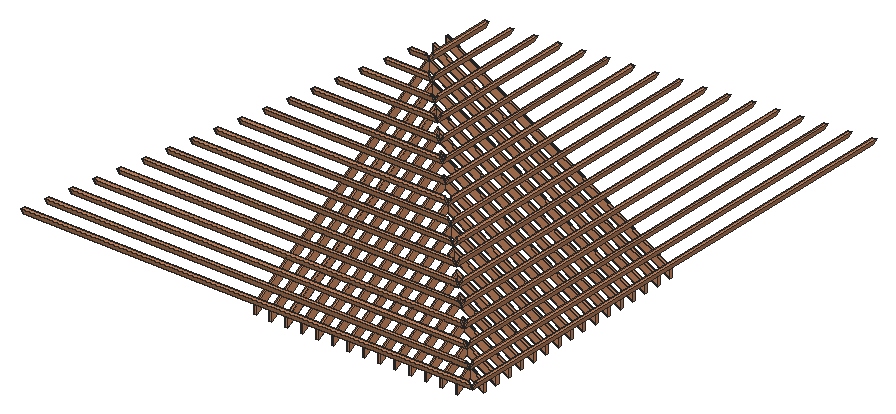
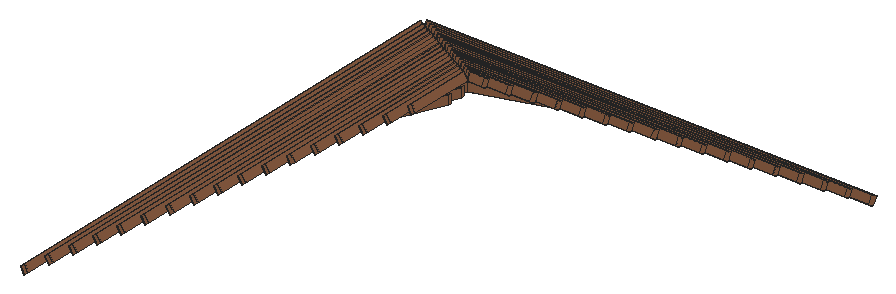
# SketchUp Ruby script. Lengths in millimetres.
U = 1.mm
M = Sketchup.active_model
def pt(a) = Geom::Point3d.new(a.map { |v| v * U })
def face(e, loops, mat)
  f = e.add_face(loops[0].map { |a| pt(a) })
  loops[1..].each { |l| e.add_face(l.map { |a| pt(a) }).erase! }
  f.material = f.back_material = mat if mat
  f
end
# faces: each face lists its corners as indices into pts; further lists are holes
def faces(e, pts, list, mat = nil) = list.each { |f| face(e, (f[0].is_a?(Array) ? f : [f]).map { |l| l.map { |i| pts[i] } }, mat) }
# xy, xz, yz: faces in a plane at the given z, y or x. An outline is a flat list of corners, or four numbers for a rectangle; further outlines are holes
def ring(l) = l.size == 4 ? [[l[0], l[1]], [l[2], l[1]], [l[2], l[3]], [l[0], l[3]]] : l.each_slice(2).to_a
def flat(e, list, mat, &to3) = list.each { |f| face(e, (f[0].is_a?(Array) ? f : [f]).map { |l| ring(l).map { |u, v| to3.(u, v) } }, mat) }
def xy(e, z, list, mat = nil) = flat(e, list, mat) { |x, y| [x, y, z] }
def xz(e, y, list, mat = nil) = flat(e, list, mat) { |x, z| [x, y, z] }
def yz(e, x, list, mat = nil) = flat(e, list, mat) { |y, z| [x, y, z] }
def lines(e, pts, list) = list.each { |a, b| e.add_line(pt(pts[a]), pt(pts[b])) }
# prism: a flat outline (further loops are holes) pulled along v
def prism(e, loops, v, mat = nil)
  f = face(e, loops, mat); d = Geom::Vector3d.new(v.map { |x| x * U })
  f.pushpull(f.normal.samedirection?(d) ? d.length : -d.length)
end
def box(e, o, s, mat = nil) = prism(e, [[o, [o[0] + s[0], o[1], o[2]], [o[0] + s[0], o[1] + s[1], o[2]], [o[0], o[1] + s[1], o[2]]]], [0, 0, s[2]], mat)
def at(x, y, z, deg = 0) = Geom::Transformation.translation(pt([x, y, z])) * Geom::Transformation.rotation(ORIGIN, Z_AXIS, deg.degrees)
def axes(o, x, y, z) = Geom::Transformation.new([*x, 0, *y, 0, *z, 0, *pt(o).to_a, 1])
def part(name) = M.definitions.add(name)
# library, detail: a bought-in or finely detailed component or shape, given as its bounding box
def library(name, o, s) = part(name).tap { |d| box(d.entities, o, s) }
def detail(e, o, s) = box(e.add_group.entities, o, s)
def put(e, d, t, mat = nil) = e.add_instance(d, t).tap { |i| i.material = mat if mat }
def group(e, t, mat = nil) = e.add_group.tap { |g| g.transformation = t; g.material = mat if mat }.entities
root = M.entities
M.materials.add("[Wood Veneer 02]").color = [190, 128, 91]
c1 = part("Group243\#1")
prism(c1.entities,[[[4410,-2546.1,0],[-4410,-2546.1,0],[-4365.8,-2495.1,0],[4365.8,-2495.1,0]]],[0,0,152])
c2 = part("Group244\#1")
prism(c2.entities,[[[4145.9,-2241.1,0],[-4145.9,-2241.1,0],[-4101.7,-2190.1,0],[4101.7,-2190.1,0]]],[0,0,152])
c3 = part("Group245\#1")
prism(c3.entities,[[[3881.7,-1936.1,0],[-3881.7,-1936.1,0],[-3837.6,-1885.1,0],[3837.6,-1885.1,0]]],[0,0,152])
c4 = part("Group246\#1")
prism(c4.entities,[[[-3573.4,-1580.1,0],[3573.4,-1580.1,0],[3617.6,-1631.1,0],[-3617.6,-1631.1,0]]],[0,0,152])
c5 = part("Group247\#1")
prism(c5.entities,[[[-3309.3,-1275.1,0],[3309.3,-1275.1,0],[3353.4,-1326.1,0],[-3353.4,-1326.1,0]]],[0,0,152])
c6 = part("Group248\#1")
prism(c6.entities,[[[3089.3,-1021.1,0],[-3089.3,-1021.1,0],[-3045.1,-970.1,0],[3045.1,-970.1,0]]],[0,0,152])
c7 = part("Group249\#1")
prism(c7.entities,[[[-2781,-665.1,0],[2781,-665.1,0],[2825.2,-716.1,0],[-2825.2,-716.1,0]]],[0,0,152])
c8 = part("Group250\#1")
prism(c8.entities,[[[-2516.9,-360.1,0],[2516.9,-360.1,0],[2561,-411.1,0],[-2561,-411.1,0]]],[0,0,152])
c9 = part("Group251\#1")
prism(c9.entities,[[[-2252.7,-55.1,0],[2252.7,-55.1,0],[2296.9,-106.1,0],[-2296.9,-106.1,0]]],[0,0,152])
c10 = part("Group252\#1")
prism(c10.entities,[[[2032.8,198.9,0],[-2032.8,198.9,0],[-1988.6,249.9,0],[1988.6,249.9,0]]],[0,0,152])
c11 = part("Group253\#1")
prism(c11.entities,[[[1768.6,503.9,0],[-1768.6,503.9,0],[-1724.5,554.9,0],[1724.5,554.9,0]]],[0,0,152])
c12 = part("Group254\#1")
prism(c12.entities,[[[1504.5,808.9,0],[-1504.5,808.9,0],[-1460.3,859.9,0],[1460.3,859.9,0]]],[0,0,152])
c13 = part("Group255\#1")
prism(c13.entities,[[[-1196.2,1164.9,0],[1196.2,1164.9,0],[1240.3,1113.9,0],[-1240.3,1113.9,0]]],[0,0,152])
c14 = part("Group256\#1")
prism(c14.entities,[[[-932,1469.9,0],[932,1469.9,0],[976.2,1418.9,0],[-976.2,1418.9,0]]],[0,0,152])
c15 = part("Group257\#1")
prism(c15.entities,[[[712.1,1723.9,0],[-712.1,1723.9,0],[-667.9,1774.9,0],[667.9,1774.9,0]]],[0,0,152])
c16 = part("Group258\#1")
prism(c16.entities,[[[447.9,2028.9,0],[-447.9,2028.9,0],[-403.8,2079.9,0],[403.8,2079.9,0]]],[0,0,152])
c17 = part("Group259\#1")
prism(c17.entities,[[[183.8,2333.9,0],[-183.8,2333.9,0],[-139.6,2384.9,0],[139.6,2384.9,0]]],[0,0,152])
c18 = part("Group241\#2")
put(c18.entities,c1,at(0,0,0))
put(c18.entities,c2,at(0,0,0))
put(c18.entities,c3,at(0,0,0))
put(c18.entities,c4,at(0,0,0))
put(c18.entities,c5,at(0,0,0))
put(c18.entities,c6,at(0,0,0))
put(c18.entities,c7,at(0,0,0))
put(c18.entities,c8,at(0,0,0))
put(c18.entities,c9,at(0,0,0))
put(c18.entities,c10,at(0,0,0))
put(c18.entities,c11,at(0,0,0))
put(c18.entities,c12,at(0,0,0))
put(c18.entities,c13,at(0,0,0))
put(c18.entities,c14,at(0,0,0))
put(c18.entities,c15,at(0,0,0))
put(c18.entities,c16,at(0,0,0))
put(c18.entities,c17,at(0,0,0))
c19 = part("Group241\#1")
xy(c19.entities,0,[[-4960,-4295.5,-4901.1,-4244.5,0,-4244.5,0,-4295.5]])
xy(c19.entities,152,[[-5047.8,-4295.5,-87.8,-4295.5,-87.8,-4244.5,-4988.9,-4244.5]])
xz(c19.entities,-4295.5,[[-4960,0,0,0,-87.8,152,-5047.8,152]])
xz(c19.entities,-4244.5,[[-4901.1,0,-4988.9,152,-87.8,152,0,0]])
p = [[-4901.1,-4244.5,0],[-4960,-4295.5,0],[-5047.8,-4295.5,152],[-4988.9,-4244.5,152],[0,-4295.5,0],[0,-4244.5,0],
  [-87.8,-4244.5,152],[-87.8,-4295.5,152]]
faces(c19.entities,p,[[0,1,2,3],[4,5,6,7]])
c20 = part("Group239\#1")
xy(c20.entities,0,[[-4607.8,-3990.5,-4548.9,-3939.5,0,-3939.5,0,-3990.5]])
xy(c20.entities,152,[[-4695.6,-3990.5,-87.8,-3990.5,-87.8,-3939.5,-4636.7,-3939.5]])
xz(c20.entities,-3990.5,[[-4607.8,0,0,0,-87.8,152,-4695.6,152]])
xz(c20.entities,-3939.5,[[-4548.9,0,-4636.7,152,-87.8,152,0,0]])
p = [[-4636.7,-3939.5,152],[-4548.9,-3939.5,0],[-4607.8,-3990.5,0],[-4695.6,-3990.5,152],[0,-3939.5,0],[-87.8,-3939.5,152],
  [-87.8,-3990.5,152],[0,-3990.5,0]]
faces(c20.entities,p,[[0,1,2,3],[4,5,6,7]])
c21 = part("Group237\#1")
xy(c21.entities,0,[[-4255.6,-3685.5,-4196.8,-3634.5,0,-3634.5,0,-3685.5]])
xy(c21.entities,152,[[-4343.4,-3685.5,-87.8,-3685.5,-87.8,-3634.5,-4284.5,-3634.5]])
xz(c21.entities,-3685.5,[[-4255.6,0,0,0,-87.8,152,-4343.4,152]])
xz(c21.entities,-3634.5,[[-4196.8,0,-4284.5,152,-87.8,152,0,0]])
p = [[-4284.5,-3634.5,152],[-4196.8,-3634.5,0],[-4255.6,-3685.5,0],[-4343.4,-3685.5,152],[0,-3634.5,0],[-87.8,-3634.5,152],
  [-87.8,-3685.5,152],[0,-3685.5,0]]
faces(c21.entities,p,[[0,1,2,3],[4,5,6,7]])
c22 = part("Group235\#1")
xy(c22.entities,0,[[-3903.5,-3380.5,-3844.6,-3329.5,0,-3329.5,0,-3380.5]])
xy(c22.entities,152,[[-3991.2,-3380.5,-87.8,-3380.5,-87.8,-3329.5,-3932.3,-3329.5]])
xz(c22.entities,-3380.5,[[-3903.5,0,0,0,-87.8,152,-3991.2,152]])
xz(c22.entities,-3329.5,[[-3844.6,0,-3932.3,152,-87.8,152,0,0]])
p = [[-3991.2,-3380.5,152],[-3932.3,-3329.5,152],[-3844.6,-3329.5,0],[-3903.5,-3380.5,0],[-87.8,-3329.5,152],[-87.8,-3380.5,152],
  [0,-3380.5,0],[0,-3329.5,0]]
faces(c22.entities,p,[[0,1,2,3],[4,5,6,7]])
c23 = part("Group233\#1")
xy(c23.entities,0,[[-3551.3,-3075.5,-3492.4,-3024.5,0,-3024.5,0,-3075.5]])
xy(c23.entities,152,[[-3639,-3075.5,-87.8,-3075.5,-87.8,-3024.5,-3580.1,-3024.5]])
xz(c23.entities,-3075.5,[[-3551.3,0,0,0,-87.8,152,-3639,152]])
xz(c23.entities,-3024.5,[[-3492.4,0,-3580.1,152,-87.8,152,0,0]])
p = [[-3492.4,-3024.5,0],[-3551.3,-3075.5,0],[-3639,-3075.5,152],[-3580.1,-3024.5,152],[0,-3075.5,0],[0,-3024.5,0],
  [-87.8,-3024.5,152],[-87.8,-3075.5,152]]
faces(c23.entities,p,[[0,1,2,3],[4,5,6,7]])
c24 = part("Group231\#1")
xy(c24.entities,0,[[-3199.1,-2770.5,-3140.2,-2719.5,0,-2719.5,0,-2770.5]])
xy(c24.entities,152,[[-3286.9,-2770.5,-87.8,-2770.5,-87.8,-2719.5,-3228,-2719.5]])
xz(c24.entities,-2770.5,[[-3199.1,0,0,0,-87.8,152,-3286.9,152]])
xz(c24.entities,-2719.5,[[-3140.2,0,-3228,152,-87.8,152,0,0]])
p = [[-3199.1,-2770.5,0],[-3286.9,-2770.5,152],[-3228,-2719.5,152],[-3140.2,-2719.5,0],[-87.8,-2770.5,152],[0,-2770.5,0],
  [0,-2719.5,0],[-87.8,-2719.5,152]]
faces(c24.entities,p,[[0,1,2,3],[4,5,6,7]])
c25 = part("Group229\#1")
xy(c25.entities,0,[[-2846.9,-2465.5,-2788,-2414.5,0,-2414.5,0,-2465.5]])
xy(c25.entities,152,[[-2934.7,-2465.5,-87.8,-2465.5,-87.8,-2414.5,-2875.8,-2414.5]])
xz(c25.entities,-2465.5,[[-2846.9,0,0,0,-87.8,152,-2934.7,152]])
xz(c25.entities,-2414.5,[[-2788,0,-2875.8,152,-87.8,152,0,0]])
p = [[-2846.9,-2465.5,0],[-2934.7,-2465.5,152],[-2875.8,-2414.5,152],[-2788,-2414.5,0],[-87.8,-2465.5,152],[0,-2465.5,0],
  [0,-2414.5,0],[-87.8,-2414.5,152]]
faces(c25.entities,p,[[0,1,2,3],[4,5,6,7]])
c26 = part("Group90\#1")
prism(c26.entities,[[[0,-5222.6,0],[-5092.2,-5222.6,0],[-5180.2,-5222.6,152.4],[-88,-5222.6,152.4]]],[0,-50.8,0])
c27 = part("Group92\#1")
prism(c27.entities,[[[-5180.2,-4917.8,152.4],[-88,-4917.8,152.4],[0,-4917.8,0],[-5092.2,-4917.8,0]]],[0,-50.8,0])
c28 = part("Group88\#1")
xy(c28.entities,0,[[-4898,-5578.2,-4956.7,-5527.4,0,-5527.4,0,-5578.2]])
xy(c28.entities,152.4,[[-4986,-5578.2,-88,-5578.2,-88,-5527.4,-5044.7,-5527.4]])
xz(c28.entities,-5578.2,[[-4898,0,0,0,-88,152.4,-4986,152.4]])
xz(c28.entities,-5527.4,[[-4956.7,0,-5044.7,152.4,-88,152.4,0,0]])
p = [[-4956.7,-5527.4,0],[-4898,-5578.2,0],[-4986,-5578.2,152.4],[-5044.7,-5527.4,152.4],[0,-5578.2,0],[0,-5527.4,0],
  [-88,-5527.4,152.4],[-88,-5578.2,152.4]]
faces(c28.entities,p,[[0,1,2,3],[4,5,6,7]])
c29 = part("Group227\#1")
xy(c29.entities,0,[[-2494.7,-2160.5,-2435.8,-2109.5,0,-2109.5,0,-2160.5]])
xy(c29.entities,152,[[-2582.5,-2160.5,-87.8,-2160.5,-87.8,-2109.5,-2523.6,-2109.5]])
xz(c29.entities,-2160.5,[[-2494.7,0,0,0,-87.8,152,-2582.5,152]])
xz(c29.entities,-2109.5,[[-2435.8,0,-2523.6,152,-87.8,152,0,0]])
p = [[-2523.6,-2109.5,152],[-2435.8,-2109.5,0],[-2494.7,-2160.5,0],[-2582.5,-2160.5,152],[0,-2109.5,0],[-87.8,-2109.5,152],
  [-87.8,-2160.5,152],[0,-2160.5,0]]
faces(c29.entities,p,[[0,1,2,3],[4,5,6,7]])
c30 = part("Group95\#1")
prism(c30.entities,[[[-4866,-2495.3,0],[4866,-2495.3,0],[4910,-2546.1,0],[-4910,-2546.1,0]]],[0,0,152.4])
c31 = part("Group96\#1")
prism(c31.entities,[[[4646,-2241.3,0],[-4646,-2241.3,0],[-4602,-2190.5,0],[4602,-2190.5,0]]],[0,0,152.4])
c32 = part("Group97\#1")
prism(c32.entities,[[[4382.1,-1936.5,0],[-4382.1,-1936.5,0],[-4338.1,-1885.7,0],[4338.1,-1885.7,0]]],[0,0,152.4])
c33 = part("Group98\#1")
prism(c33.entities,[[[4118.1,-1631.7,0],[-4118.1,-1631.7,0],[-4074.1,-1580.9,0],[4074.1,-1580.9,0]]],[0,0,152.4])
c34 = part("Group99\#1")
prism(c34.entities,[[[3854.1,-1326.9,0],[-3854.1,-1326.9,0],[-3810.1,-1276.1,0],[3810.1,-1276.1,0]]],[0,0,152.4])
c35 = part("Group100\#1")
prism(c35.entities,[[[3590.2,-1022.1,0],[-3590.2,-1022.1,0],[-3546.2,-971.3,0],[3546.2,-971.3,0]]],[0,0,152.4])
c36 = part("Group101\#1")
prism(c36.entities,[[[3326.2,-717.3,0],[-3326.2,-717.3,0],[-3282.2,-666.5,0],[3282.2,-666.5,0]]],[0,0,152.4])
c37 = part("Group102\#1")
prism(c37.entities,[[[3062.2,-412.5,0],[-3062.2,-412.5,0],[-3018.3,-361.7,0],[3018.3,-361.7,0]]],[0,0,152.4])
c38 = part("Group103\#1")
prism(c38.entities,[[[2798.3,-107.7,0],[-2798.3,-107.7,0],[-2754.3,-56.9,0],[2754.3,-56.9,0]]],[0,0,152.4])
c39 = part("Group104\#1")
prism(c39.entities,[[[2534.3,197.1,0],[-2534.3,197.1,0],[-2490.3,247.9,0],[2490.3,247.9,0]]],[0,0,152.4])
c40 = part("Group105\#1")
prism(c40.entities,[[[2270.4,501.9,0],[-2270.4,501.9,0],[-2226.4,552.7,0],[2226.4,552.7,0]]],[0,0,152.4])
c41 = part("Group106\#1")
prism(c41.entities,[[[2006.4,806.7,0],[-2006.4,806.7,0],[-1962.4,857.5,0],[1962.4,857.5,0]]],[0,0,152.4])
c42 = part("Group107\#1")
prism(c42.entities,[[[1742.4,1111.5,0],[-1742.4,1111.5,0],[-1698.4,1162.3,0],[1698.4,1162.3,0]]],[0,0,152.4])
c43 = part("Group108\#1")
prism(c43.entities,[[[1478.5,1416.3,0],[-1478.5,1416.3,0],[-1434.5,1467.1,0],[1434.5,1467.1,0]]],[0,0,152.4])
c44 = part("Group109\#1")
prism(c44.entities,[[[-1170.5,1771.9,0],[1170.5,1771.9,0],[1214.5,1721.1,0],[-1214.5,1721.1,0]]],[0,0,152.4])
c45 = part("Group110\#1")
prism(c45.entities,[[[950.5,2025.9,0],[-950.5,2025.9,0],[-906.5,2076.7,0],[906.5,2076.7,0]]],[0,0,152.4])
c46 = part("Group111\#1")
prism(c46.entities,[[[686.6,2330.7,0],[-686.6,2330.7,0],[-642.6,2381.5,0],[642.6,2381.5,0]]],[0,0,152.4])
c47 = part("Group93\#2")
put(c47.entities,c30,at(0,0,0))
put(c47.entities,c31,at(0,0,0))
put(c47.entities,c32,at(0,0,0))
put(c47.entities,c33,at(0,0,0))
put(c47.entities,c34,at(0,0,0))
put(c47.entities,c35,at(0,0,0))
put(c47.entities,c36,at(0,0,0))
put(c47.entities,c37,at(0,0,0))
put(c47.entities,c38,at(0,0,0))
put(c47.entities,c39,at(0,0,0))
put(c47.entities,c40,at(0,0,0))
put(c47.entities,c41,at(0,0,0))
put(c47.entities,c42,at(0,0,0))
put(c47.entities,c43,at(0,0,0))
put(c47.entities,c44,at(0,0,0))
put(c47.entities,c45,at(0,0,0))
put(c47.entities,c46,at(0,0,0))
c48 = part("Group86\#1")
xy(c48.entities,0,[[-4546.1,-5883,-4604.7,-5832.2,0,-5832.2,0,-5883]])
xy(c48.entities,152.4,[[-4634,-5883,-88,-5883,-88,-5832.2,-4692.7,-5832.2]])
xz(c48.entities,-5883,[[-4546.1,0,0,0,-88,152.4,-4634,152.4]])
xz(c48.entities,-5832.2,[[-4604.7,0,-4692.7,152.4,-88,152.4,0,0]])
p = [[-4604.7,-5832.2,0],[-4546.1,-5883,0],[-4634,-5883,152.4],[-4692.7,-5832.2,152.4],[0,-5883,0],[0,-5832.2,0],
  [-88,-5832.2,152.4],[-88,-5883,152.4]]
faces(c48.entities,p,[[0,1,2,3],[4,5,6,7]])
c49 = part("Group84\#1")
xy(c49.entities,0,[[-4194.1,-6187.8,-4252.8,-6137,0,-6137,0,-6187.8]])
xy(c49.entities,152.4,[[-4282.1,-6187.8,-88,-6187.8,-88,-6137,-4340.8,-6137]])
xz(c49.entities,-6187.8,[[-4194.1,0,0,0,-88,152.4,-4282.1,152.4]])
xz(c49.entities,-6137,[[-4252.8,0,-4340.8,152.4,-88,152.4,0,0]])
p = [[-4282.1,-6187.8,152.4],[-4340.8,-6137,152.4],[-4252.8,-6137,0],[-4194.1,-6187.8,0],[-88,-6137,152.4],[-88,-6187.8,152.4],
  [0,-6187.8,0],[0,-6137,0]]
faces(c49.entities,p,[[0,1,2,3],[4,5,6,7]])
c50 = part("Group225\#1")
xy(c50.entities,0,[[-2142.5,-1855.5,-2083.7,-1804.5,0,-1804.5,0,-1855.5]])
xy(c50.entities,152,[[-2230.3,-1855.5,-87.8,-1855.5,-87.8,-1804.5,-2171.4,-1804.5]])
xz(c50.entities,-1855.5,[[-2142.5,0,0,0,-87.8,152,-2230.3,152]])
xz(c50.entities,-1804.5,[[-2083.7,0,-2171.4,152,-87.8,152,0,0]])
p = [[-2083.7,-1804.5,0],[-2142.5,-1855.5,0],[-2230.3,-1855.5,152],[-2171.4,-1804.5,152],[0,-1855.5,0],[0,-1804.5,0],
  [-87.8,-1804.5,152],[-87.8,-1855.5,152]]
faces(c50.entities,p,[[0,1,2,3],[4,5,6,7]])
c51 = part("Group82\#1")
xy(c51.entities,0,[[-3842.2,-6492.6,-3900.8,-6441.8,0,-6441.8,0,-6492.6]])
xy(c51.entities,152.4,[[-3930.1,-6492.6,-88,-6492.6,-88,-6441.8,-3988.8,-6441.8]])
xz(c51.entities,-6492.6,[[-3842.2,0,0,0,-88,152.4,-3930.1,152.4]])
xz(c51.entities,-6441.8,[[-3900.8,0,-3988.8,152.4,-88,152.4,0,0]])
p = [[-3900.8,-6441.8,0],[-3842.2,-6492.6,0],[-3930.1,-6492.6,152.4],[-3988.8,-6441.8,152.4],[0,-6492.6,0],[0,-6441.8,0],
  [-88,-6441.8,152.4],[-88,-6492.6,152.4]]
faces(c51.entities,p,[[0,1,2,3],[4,5,6,7]])
c52 = part("Group80\#1")
xy(c52.entities,0,[[-3490.2,-6797.4,-3548.9,-6746.6,0,-6746.6,0,-6797.4]])
xy(c52.entities,152.4,[[-3578.2,-6797.4,-88,-6797.4,-88,-6746.6,-3636.8,-6746.6]])
xz(c52.entities,-6797.4,[[-3490.2,0,0,0,-88,152.4,-3578.2,152.4]])
xz(c52.entities,-6746.6,[[-3548.9,0,-3636.8,152.4,-88,152.4,0,0]])
p = [[-3548.9,-6746.6,0],[-3490.2,-6797.4,0],[-3578.2,-6797.4,152.4],[-3636.8,-6746.6,152.4],[0,-6797.4,0],[0,-6746.6,0],
  [-88,-6746.6,152.4],[-88,-6797.4,152.4]]
faces(c52.entities,p,[[0,1,2,3],[4,5,6,7]])
c53 = part("Group223\#1")
xy(c53.entities,0,[[-1790.4,-1550.5,-1731.5,-1499.5,0,-1499.5,0,-1550.5]])
xy(c53.entities,152,[[-1878.1,-1550.5,-87.8,-1550.5,-87.8,-1499.5,-1819.2,-1499.5]])
xz(c53.entities,-1550.5,[[-1790.4,0,0,0,-87.8,152,-1878.1,152]])
xz(c53.entities,-1499.5,[[-1731.5,0,-1819.2,152,-87.8,152,0,0]])
p = [[-1731.5,-1499.5,0],[-1790.4,-1550.5,0],[-1878.1,-1550.5,152],[-1819.2,-1499.5,152],[0,-1550.5,0],[0,-1499.5,0],
  [-87.8,-1499.5,152],[-87.8,-1550.5,152]]
faces(c53.entities,p,[[0,1,2,3],[4,5,6,7]])
c54 = part("Group78\#1")
xy(c54.entities,0,[[-3138.2,-7102.2,-3196.9,-7051.4,0,-7051.4,0,-7102.2]])
xy(c54.entities,152.4,[[-3226.2,-7102.2,-88,-7102.2,-88,-7051.4,-3284.9,-7051.4]])
xz(c54.entities,-7102.2,[[-3138.2,0,0,0,-88,152.4,-3226.2,152.4]])
xz(c54.entities,-7051.4,[[-3196.9,0,-3284.9,152.4,-88,152.4,0,0]])
p = [[-3196.9,-7051.4,0],[-3138.2,-7102.2,0],[-3226.2,-7102.2,152.4],[-3284.9,-7051.4,152.4],[0,-7102.2,0],[0,-7051.4,0],
  [-88,-7051.4,152.4],[-88,-7102.2,152.4]]
faces(c54.entities,p,[[0,1,2,3],[4,5,6,7]])
c55 = part("Group76\#1")
xy(c55.entities,0,[[-2786.3,-7407,-2845,-7356.2,0,-7356.2,0,-7407]])
xy(c55.entities,152.4,[[-2874.3,-7407,-88,-7407,-88,-7356.2,-2932.9,-7356.2]])
xz(c55.entities,-7407,[[-2786.3,0,0,0,-88,152.4,-2874.3,152.4]])
xz(c55.entities,-7356.2,[[-2845,0,-2932.9,152.4,-88,152.4,0,0]])
p = [[-2845,-7356.2,0],[-2786.3,-7407,0],[-2874.3,-7407,152.4],[-2932.9,-7356.2,152.4],[0,-7407,0],[0,-7356.2,0],
  [-88,-7356.2,152.4],[-88,-7407,152.4]]
faces(c55.entities,p,[[0,1,2,3],[4,5,6,7]])
c56 = part("Group221\#1")
xy(c56.entities,0,[[-1438.2,-1245.5,-1379.3,-1194.5,0,-1194.5,0,-1245.5]])
xy(c56.entities,152,[[-1525.9,-1245.5,-87.8,-1245.5,-87.8,-1194.5,-1467,-1194.5]])
xz(c56.entities,-1245.5,[[-1438.2,0,0,0,-87.8,152,-1525.9,152]])
xz(c56.entities,-1194.5,[[-1379.3,0,-1467,152,-87.8,152,0,0]])
p = [[-1467,-1194.5,152],[-1379.3,-1194.5,0],[-1438.2,-1245.5,0],[-1525.9,-1245.5,152],[0,-1194.5,0],[-87.8,-1194.5,152],
  [-87.8,-1245.5,152],[0,-1245.5,0]]
faces(c56.entities,p,[[0,1,2,3],[4,5,6,7]])
c57 = part("Group74\#1")
xy(c57.entities,0,[[-2434.3,-7711.8,-2493,-7661,0,-7661,0,-7711.8]])
xy(c57.entities,152.4,[[-2522.3,-7711.8,-88,-7711.8,-88,-7661,-2581,-7661]])
xz(c57.entities,-7711.8,[[-2434.3,0,0,0,-88,152.4,-2522.3,152.4]])
xz(c57.entities,-7661,[[-2493,0,-2581,152.4,-88,152.4,0,0]])
p = [[-2434.3,-7711.8,0],[-2522.3,-7711.8,152.4],[-2581,-7661,152.4],[-2493,-7661,0],[-88,-7711.8,152.4],[0,-7711.8,0],
  [0,-7661,0],[-88,-7661,152.4]]
faces(c57.entities,p,[[0,1,2,3],[4,5,6,7]])
c58 = part("Group72\#1")
xy(c58.entities,0,[[-2082.4,-8016.6,-2141,-7965.8,0,-7965.8,0,-8016.6]])
xy(c58.entities,152.4,[[-2170.4,-8016.6,-88,-8016.6,-88,-7965.8,-2229,-7965.8]])
xz(c58.entities,-8016.6,[[-2082.4,0,0,0,-88,152.4,-2170.4,152.4]])
xz(c58.entities,-7965.8,[[-2141,0,-2229,152.4,-88,152.4,0,0]])
p = [[-2170.4,-8016.6,152.4],[-2229,-7965.8,152.4],[-2141,-7965.8,0],[-2082.4,-8016.6,0],[-88,-7965.8,152.4],[-88,-8016.6,152.4],
  [0,-8016.6,0],[0,-7965.8,0]]
faces(c58.entities,p,[[0,1,2,3],[4,5,6,7]])
c59 = part("Group219\#1")
xy(c59.entities,0,[[-1086,-940.5,-1027.1,-889.5,0,-889.5,0,-940.5]])
xy(c59.entities,152,[[-1173.8,-940.5,-87.8,-940.5,-87.8,-889.5,-1114.9,-889.5]])
xz(c59.entities,-940.5,[[-1086,0,0,0,-87.8,152,-1173.8,152]])
xz(c59.entities,-889.5,[[-1027.1,0,-1114.9,152,-87.8,152,0,0]])
p = [[-1114.9,-889.5,152],[-1027.1,-889.5,0],[-1086,-940.5,0],[-1173.8,-940.5,152],[0,-889.5,0],[-87.8,-889.5,152],
  [-87.8,-940.5,152],[0,-940.5,0]]
faces(c59.entities,p,[[0,1,2,3],[4,5,6,7]])
c60 = part("Group70\#1")
xy(c60.entities,0,[[-1730.4,-8321.4,-1789.1,-8270.6,0,-8270.6,0,-8321.4]])
xy(c60.entities,152.4,[[-1818.4,-8321.4,-88,-8321.4,-88,-8270.6,-1877.1,-8270.6]])
xz(c60.entities,-8321.4,[[-1730.4,0,0,0,-88,152.4,-1818.4,152.4]])
xz(c60.entities,-8270.6,[[-1789.1,0,-1877.1,152.4,-88,152.4,0,0]])
p = [[-1730.4,-8321.4,0],[-1818.4,-8321.4,152.4],[-1877.1,-8270.6,152.4],[-1789.1,-8270.6,0],[-88,-8321.4,152.4],[0,-8321.4,0],
  [0,-8270.6,0],[-88,-8270.6,152.4]]
faces(c60.entities,p,[[0,1,2,3],[4,5,6,7]])
c61 = part("Group68\#1")
xy(c61.entities,0,[[-1378.5,-8626.2,-1437.1,-8575.4,0,-8575.4,0,-8626.2]])
xy(c61.entities,152.4,[[-1466.5,-8626.2,-88,-8626.2,-88,-8575.4,-1525.1,-8575.4]])
xz(c61.entities,-8626.2,[[-1378.5,0,0,0,-88,152.4,-1466.5,152.4]])
xz(c61.entities,-8575.4,[[-1437.1,0,-1525.1,152.4,-88,152.4,0,0]])
p = [[-1525.1,-8575.4,152.4],[-1437.1,-8575.4,0],[-1378.5,-8626.2,0],[-1466.5,-8626.2,152.4],[0,-8575.4,0],[-88,-8575.4,152.4],
  [-88,-8626.2,152.4],[0,-8626.2,0]]
faces(c61.entities,p,[[0,1,2,3],[4,5,6,7]])
c62 = part("Group217\#1")
xy(c62.entities,0,[[-733.8,-635.5,-674.9,-584.5,0,-584.5,0,-635.5]])
xy(c62.entities,152,[[-821.6,-635.5,-87.8,-635.5,-87.8,-584.5,-762.7,-584.5]])
xz(c62.entities,-635.5,[[-733.8,0,0,0,-87.8,152,-821.6,152]])
xz(c62.entities,-584.5,[[-674.9,0,-762.7,152,-87.8,152,0,0]])
p = [[-733.8,-635.5,0],[-821.6,-635.5,152],[-762.7,-584.5,152],[-674.9,-584.5,0],[-87.8,-635.5,152],[0,-635.5,0],
  [0,-584.5,0],[-87.8,-584.5,152]]
faces(c62.entities,p,[[0,1,2,3],[4,5,6,7]])
c63 = part("Group66\#1")
xy(c63.entities,0,[[-1026.5,-8931,-1085.2,-8880.2,0,-8880.2,0,-8931]])
xy(c63.entities,152.4,[[-1114.5,-8931,-88,-8931,-88,-8880.2,-1173.2,-8880.2]])
xz(c63.entities,-8931,[[-1026.5,0,0,0,-88,152.4,-1114.5,152.4]])
xz(c63.entities,-8880.2,[[-1085.2,0,-1173.2,152.4,-88,152.4,0,0]])
p = [[-1085.2,-8880.2,0],[-1026.5,-8931,0],[-1114.5,-8931,152.4],[-1173.2,-8880.2,152.4],[0,-8931,0],[0,-8880.2,0],
  [-88,-8880.2,152.4],[-88,-8931,152.4]]
faces(c63.entities,p,[[0,1,2,3],[4,5,6,7]])
c64 = part("Group64\#1")
xy(c64.entities,0,[[-674.6,-9235.8,-733.2,-9185,0,-9185,0,-9235.8]])
xy(c64.entities,152.4,[[-762.6,-9235.8,-88,-9235.8,-88,-9185,-821.2,-9185]])
xz(c64.entities,-9235.8,[[-674.6,0,0,0,-88,152.4,-762.6,152.4]])
xz(c64.entities,-9185,[[-733.2,0,-821.2,152.4,-88,152.4,0,0]])
p = [[-733.2,-9185,0],[-674.6,-9235.8,0],[-762.6,-9235.8,152.4],[-821.2,-9185,152.4],[0,-9235.8,0],[0,-9185,0],
  [-88,-9185,152.4],[-88,-9235.8,152.4]]
faces(c64.entities,p,[[0,1,2,3],[4,5,6,7]])
c65 = part("Group215\#1")
xy(c65.entities,0,[[-381.6,-330.5,-322.7,-279.5,0,-279.5,0,-330.5]])
xy(c65.entities,152,[[-469.4,-330.5,-87.8,-330.5,-87.8,-279.5,-410.5,-279.5]])
xz(c65.entities,-330.5,[[-381.6,0,0,0,-87.8,152,-469.4,152]])
xz(c65.entities,-279.5,[[-322.7,0,-410.5,152,-87.8,152,0,0]])
p = [[-469.4,-330.5,152],[-410.5,-279.5,152],[-322.7,-279.5,0],[-381.6,-330.5,0],[-87.8,-279.5,152],[-87.8,-330.5,152],
  [0,-330.5,0],[0,-279.5,0]]
faces(c65.entities,p,[[0,1,2,3],[4,5,6,7]])
c66 = part("Group62\#1")
xy(c66.entities,0,[[-322.6,-9540.6,-381.3,-9489.8,0,-9489.8,0,-9540.6]])
xy(c66.entities,152.4,[[-410.6,-9540.6,-88,-9540.6,-88,-9489.8,-469.3,-9489.8]])
xz(c66.entities,-9540.6,[[-322.6,0,0,0,-88,152.4,-410.6,152.4]])
xz(c66.entities,-9489.8,[[-381.3,0,-469.3,152.4,-88,152.4,0,0]])
p = [[-381.3,-9489.8,0],[-322.6,-9540.6,0],[-410.6,-9540.6,152.4],[-469.3,-9489.8,152.4],[0,-9540.6,0],[0,-9489.8,0],
  [-88,-9489.8,152.4],[-88,-9540.6,152.4]]
faces(c66.entities,p,[[0,1,2,3],[4,5,6,7]])
put(root,c18,axes([5713.3,3492,4598.2],[1,0,0],[0,0.86603,0.5],[0,-0.5,0.86603]),"[Wood Veneer 02]")
put(root,c19,axes([10123.3,1287,3149.6],[0,-0.86603,-0.5],[1,0,0],[0,-0.5,0.86603]),"[Wood Veneer 02]")
put(root,c20,axes([10123.3,1287,3149.6],[0,-0.86603,-0.5],[1,0,0],[0,-0.5,0.86603]),"[Wood Veneer 02]")
put(root,c21,axes([10123.3,1287,3149.6],[0,-0.86603,-0.5],[1,0,0],[0,-0.5,0.86603]),"[Wood Veneer 02]")
put(root,c22,axes([10123.3,1287,3149.6],[0,-0.86603,-0.5],[1,0,0],[0,-0.5,0.86603]),"[Wood Veneer 02]")
put(root,c23,axes([10123.3,1287,3149.6],[0,-0.86603,-0.5],[1,0,0],[0,-0.5,0.86603]),"[Wood Veneer 02]")
put(root,c24,axes([10123.3,1287,3149.6],[0,-0.86603,-0.5],[1,0,0],[0,-0.5,0.86603]),"[Wood Veneer 02]")
put(root,c25,axes([10123.3,1287,3149.6],[0,-0.86603,-0.5],[1,0,0],[0,-0.5,0.86603]),"[Wood Veneer 02]")
put(root,c26,axes([10123.3,11107,3149.6],[0.86603,0,-0.5],[0,1,0],[0.5,0,0.86603]),"[Wood Veneer 02]")
put(root,c27,axes([10123.3,11107,3149.6],[0.86603,0,-0.5],[0,1,0],[0.5,0,0.86603]),"[Wood Veneer 02]")
put(root,c28,axes([10123.3,11107,3149.6],[0.86603,0,-0.5],[0,1,0],[0.5,0,0.86603]),"[Wood Veneer 02]")
put(root,c29,axes([10123.3,1287,3149.6],[0,-0.86603,-0.5],[1,0,0],[0,-0.5,0.86603]),"[Wood Veneer 02]")
put(root,c47,axes([7918.3,6197,4598.6],[0,1,0],[-0.86603,0,0.5],[0.5,0,0.86603]),"[Wood Veneer 02]")
put(root,c48,axes([10123.3,11107,3149.6],[0.86603,0,-0.5],[0,1,0],[0.5,0,0.86603]),"[Wood Veneer 02]")
put(root,c49,axes([10123.3,11107,3149.6],[0.86603,0,-0.5],[0,1,0],[0.5,0,0.86603]),"[Wood Veneer 02]")
put(root,c50,axes([10123.3,1287,3149.6],[0,-0.86603,-0.5],[1,0,0],[0,-0.5,0.86603]),"[Wood Veneer 02]")
put(root,c51,axes([10123.3,11107,3149.6],[0.86603,0,-0.5],[0,1,0],[0.5,0,0.86603]),"[Wood Veneer 02]")
put(root,c52,axes([10123.3,11107,3149.6],[0.86603,0,-0.5],[0,1,0],[0.5,0,0.86603]),"[Wood Veneer 02]")
put(root,c53,axes([10123.3,1287,3149.6],[0,-0.86603,-0.5],[1,0,0],[0,-0.5,0.86603]),"[Wood Veneer 02]")
put(root,c54,axes([10123.3,11107,3149.6],[0.86603,0,-0.5],[0,1,0],[0.5,0,0.86603]),"[Wood Veneer 02]")
put(root,c55,axes([10123.3,11107,3149.6],[0.86603,0,-0.5],[0,1,0],[0.5,0,0.86603]),"[Wood Veneer 02]")
put(root,c56,axes([10123.3,1287,3149.6],[0,-0.86603,-0.5],[1,0,0],[0,-0.5,0.86603]),"[Wood Veneer 02]")
put(root,c57,axes([10123.3,11107,3149.6],[0.86603,0,-0.5],[0,1,0],[0.5,0,0.86603]),"[Wood Veneer 02]")
put(root,c58,axes([10123.3,11107,3149.6],[0.86603,0,-0.5],[0,1,0],[0.5,0,0.86603]),"[Wood Veneer 02]")
put(root,c59,axes([10123.3,1287,3149.6],[0,-0.86603,-0.5],[1,0,0],[0,-0.5,0.86603]),"[Wood Veneer 02]")
put(root,c60,axes([10123.3,11107,3149.6],[0.86603,0,-0.5],[0,1,0],[0.5,0,0.86603]),"[Wood Veneer 02]")
put(root,c61,axes([10123.3,11107,3149.6],[0.86603,0,-0.5],[0,1,0],[0.5,0,0.86603]),"[Wood Veneer 02]")
put(root,c62,axes([10123.3,1287,3149.6],[0,-0.86603,-0.5],[1,0,0],[0,-0.5,0.86603]),"[Wood Veneer 02]")
put(root,c63,axes([10123.3,11107,3149.6],[0.86603,0,-0.5],[0,1,0],[0.5,0,0.86603]),"[Wood Veneer 02]")
put(root,c64,axes([10123.3,11107,3149.6],[0.86603,0,-0.5],[0,1,0],[0.5,0,0.86603]),"[Wood Veneer 02]")
put(root,c65,axes([10123.3,1287,3149.6],[0,-0.86603,-0.5],[1,0,0],[0,-0.5,0.86603]),"[Wood Veneer 02]")
put(root,c66,axes([10123.3,11107,3149.6],[0.86603,0,-0.5],[0,1,0],[0.5,0,0.86603]),"[Wood Veneer 02]")
